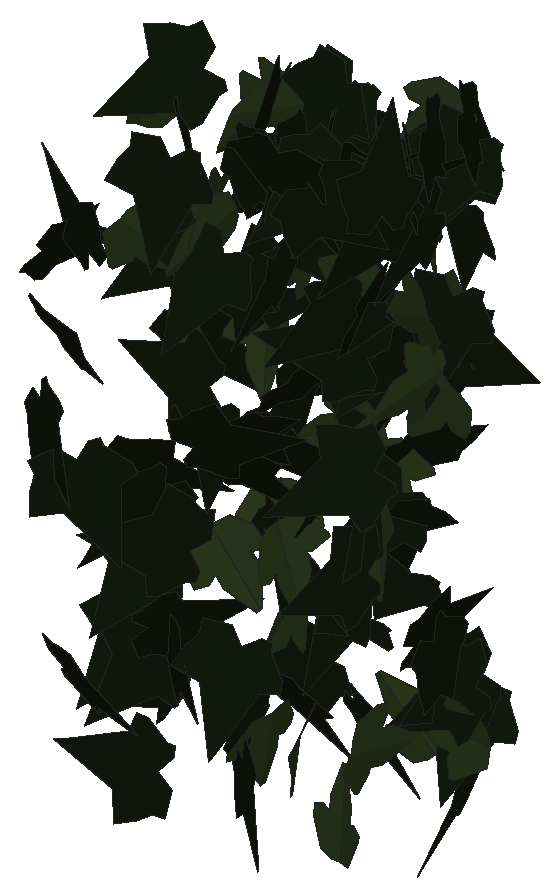
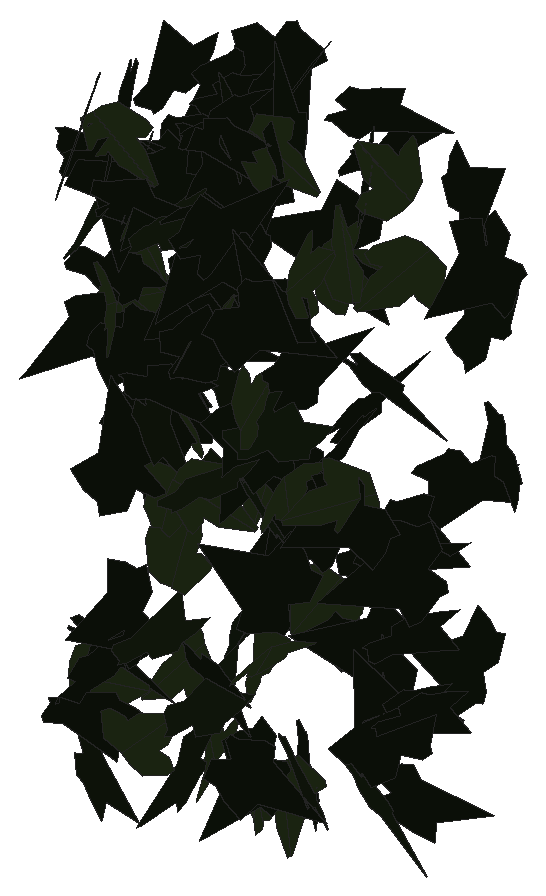
# SketchUp Ruby script. Lengths in inches.
U = 1.inch
M = Sketchup.active_model
def pt(a) = Geom::Point3d.new(a.map { |v| v * U })
def face(e, loops, mat)
  f = e.add_face(loops[0].map { |a| pt(a) })
  loops[1..].each { |l| e.add_face(l.map { |a| pt(a) }).erase! }
  f.material = f.back_material = mat if mat
  f
end
# faces: each face lists its corners as indices into pts; further lists are holes
def faces(e, pts, list, mat = nil) = list.each { |f| face(e, (f[0].is_a?(Array) ? f : [f]).map { |l| l.map { |i| pts[i] } }, mat) }
# xy, xz, yz: faces in a plane at the given z, y or x. An outline is a flat list of corners, or four numbers for a rectangle; further outlines are holes
def ring(l) = l.size == 4 ? [[l[0], l[1]], [l[2], l[1]], [l[2], l[3]], [l[0], l[3]]] : l.each_slice(2).to_a
def flat(e, list, mat, &to3) = list.each { |f| face(e, (f[0].is_a?(Array) ? f : [f]).map { |l| ring(l).map { |u, v| to3.(u, v) } }, mat) }
def xy(e, z, list, mat = nil) = flat(e, list, mat) { |x, y| [x, y, z] }
def xz(e, y, list, mat = nil) = flat(e, list, mat) { |x, z| [x, y, z] }
def yz(e, x, list, mat = nil) = flat(e, list, mat) { |y, z| [x, y, z] }
def lines(e, pts, list) = list.each { |a, b| e.add_line(pt(pts[a]), pt(pts[b])) }
# prism: a flat outline (further loops are holes) pulled along v
def prism(e, loops, v, mat = nil)
  f = face(e, loops, mat); d = Geom::Vector3d.new(v.map { |x| x * U })
  f.pushpull(f.normal.samedirection?(d) ? d.length : -d.length)
end
def box(e, o, s, mat = nil) = prism(e, [[o, [o[0] + s[0], o[1], o[2]], [o[0] + s[0], o[1] + s[1], o[2]], [o[0], o[1] + s[1], o[2]]]], [0, 0, s[2]], mat)
def at(x, y, z, deg = 0) = Geom::Transformation.translation(pt([x, y, z])) * Geom::Transformation.rotation(ORIGIN, Z_AXIS, deg.degrees)
def axes(o, x, y, z) = Geom::Transformation.new([*x, 0, *y, 0, *z, 0, *pt(o).to_a, 1])
def part(name) = M.definitions.add(name)
# library, detail: a bought-in or finely detailed component or shape, given as its bounding box
def library(name, o, s) = part(name).tap { |d| box(d.entities, o, s) }
def detail(e, o, s) = box(e.add_group.entities, o, s)
def put(e, d, t, mat = nil) = e.add_instance(d, t).tap { |i| i.material = mat if mat }
def group(e, t, mat = nil) = e.add_group.tap { |g| g.transformation = t; g.material = mat if mat }.entities
root = M.entities
M.materials.add("efeu1").color = [18, 25, 13]
M.materials.add("efeu2").color = [43, 57, 29]
c1 = part("ivyleaf_9")
p = [[1.54,2.16,1.25],[1.36,2.04,1.19],[-0.21,0.99,0.68],[-0.71,1.11,0.82],[-0.85,0.86,0.67],[-0.8,0.17,0.21],
  [-0.9,-0.01,0.1],[-0.67,-0.16,-0.02],[-0.08,-0.08,-0.05],[-0.03,-0.6,-0.4],[0.65,-0.88,-0.66],[0.83,-0.6,-0.49],
  [1.29,-0.42,-0.43],[1.8125,-0.07,-0.26],[1.21,0.44,0.15]]
faces(c1.entities,p,[[0,1,2,3,4,5,6,7,8,9,10,11,12,13,14]],"efeu1")
c2 = part("ivyleaf_10")
p = [[0,0.5,-0.03],[-0.0625,2.02,-0.43],[-0.19,2.01,-0.46],[-0.54,1.05,-0.29],[-0.52,0.625,-0.18],[-0.83,0.76,-0.28],
  [-1.16,0.64,-0.33],[-1.15,0.33,-0.24],[-0.77,-0.39,0.02],[-0.3,-0.51,0.16],[0.04,-0.48,0.23],[-0.02,2.01,-0.4375],
  [-0.06,2.01,-0.43],[0.04,-0.49,0.23],[0.67,-0.49,0.14],[1.38,0.36,-0.2],[1.375,0.51,-0.24],[0.81,0.65,-0.19],
  [0.62,0.59,-0.15],[0.6,1.09,-0.28],[0.5,1.23,-0.31]]
faces(c2.entities,p,[[0,1,2,3,4,5,6,7,8,9,10],[11,12,0,13,14,15,16,17,18,19,20]],"efeu2")
put(root,c1,axes([51.28,217.17,229.75],[0.22094,-0.00103,0.44854],[0.44724,0.03852,-0.22021],[-0.0341,0.49851,0.01794]))
put(root,c1,axes([48.23,218.1,229.92],[0.44307,-0.12316,-0.19627],[0.1976,-0.02037,0.45885],[-0.12102,-0.48417,0.03062]))
put(root,c1,axes([48.84,217.92,231.51],[0.08057,-0.14995,0.47013],[-0.25668,0.39411,0.16969],[-0.42145,-0.26869,-0.01347]))
put(root,c1,axes([48.23,218.3,224.89],[0.3039,-0.23486,0.32013],[0.24876,-0.20158,-0.38403],[0.30946,0.39269,-0.00567]))
put(root,c1,axes([47.69,218.4375,228.55],[-0.0903,-0.03685,-0.4904],[0.49111,0.01929,-0.09188],[0.02569,-0.49827,0.03271]))
put(root,c1,axes([48.37,218.33,227.95],[-0.12204,-0.31328,-0.37009],[0.14117,0.34214,-0.33617],[0.46387,-0.18654,0.00495]))
put(root,c1,axes([48.05,218.09,231.11],[0.1964,0.32583,0.32444],[0.17294,0.27456,-0.38041],[-0.42605,0.26164,-0.00485]))
put(root,c1,axes([49.52,218.77,232.61],[-0.14679,-0.47709,-0.02902],[0.00927,0.02751,-0.49916],[0.47788,-0.14708,0.00076]))
put(root,c1,axes([51.42,218.64,233.4375],[0.22565,0.22473,-0.38546],[-0.28444,-0.26034,-0.3183],[-0.34377,0.36293,0.01035]))
put(root,c1,axes([50.82,218.66,233.26],[0.32245,-0.23472,-0.30156],[-0.17593,0.25909,-0.38977],[0.33923,0.35747,0.0845]))
put(root,c1,axes([52.62,218.9,227.59],[-0.46595,0.14301,0.11152],[-0.10762,0.02941,-0.48739],[-0.14597,-0.47821,0.00337]))
put(root,c1,axes([52.4375,219.24,228.87],[-0.39221,-0.16195,0.26447],[-0.24473,-0.10025,-0.42433],[0.19047,-0.4623,-0.00063]))
put(root,c1,axes([50.27,219.27,225.45],[-0.35521,-0.31837,-0.14989],[0.12497,0.08496,-0.47662],[0.32895,-0.37606,0.01922]))
put(root,c1,axes([48.87,219.42,227.27],[-0.08262,0.06028,-0.48943],[0.11063,-0.48134,-0.07796],[-0.48056,-0.12117,0.06619]))
put(root,c1,axes([51.8,218.86,232.96],[0.06545,-0.16299,-0.46813],[-0.06779,0.46482,-0.17132],[0.49104,0.08589,0.03875]))
put(root,c1,axes([49.1,219.34,225.17],[0.0759,-0.08251,-0.48727],[0.49079,-0.04532,0.08412],[-0.05805,-0.49106,0.07411]))
put(root,c1,axes([51.66,219.46,232.93],[-0.35236,-0.30007,0.18922],[-0.13499,-0.13322,-0.46263],[0.32806,-0.37711,0.01287]))
put(root,c1,axes([48.89,219.24,223.22],[-0.26142,-0.13816,-0.4032],[-0.31821,-0.25141,0.29246],[-0.28355,0.40952,0.04352]))
put(root,c1,axes([49.23,219.47,226.5],[-0.15309,-0.06751,0.47117],[-0.43495,-0.18121,-0.16729],[0.19334,-0.46109,-0.00324]))
put(root,c2,axes([48.72,219.07,231.24],[-0.29511,-0.1897,-0.35626],[0.32293,0.15378,-0.34938],[0.24213,-0.43631,0.03175]))
put(root,c2,axes([51.08,219.17,227.41],[0.06416,0.4922,0.06023],[0.00954,0.0595,-0.49636],[-0.49577,0.06484,-0.00176]))
put(root,c1,axes([49.78,219.49,230.99],[-0.43714,-0.23622,-0.05576],[0.04885,0.0269,-0.49688],[0.23774,-0.43986,-0.00044]))
put(root,c1,axes([49.35,219.59,233.5625],[-0.38786,-0.17449,0.2629],[-0.23968,-0.10802,-0.4253],[0.20522,-0.45595,0.00015]))
put(root,c1,axes([51.91,219.02,228.42],[-0.11774,0.42278,0.23958],[-0.06777,0.22982,-0.43885],[-0.48119,-0.13581,0.00319]))
put(root,c1,axes([48.64,219.6875,224.73],[-0.28187,-0.35334,0.21378],[-0.11764,-0.17941,-0.45163],[0.39587,-0.3049,0.01801]))
put(root,c1,axes([51.02,219.6875,233.06],[0.04465,-0.04359,-0.49609],[0.31833,-0.38054,0.06209],[-0.38298,-0.32139,-0.00623]))
put(root,c2,axes([52.27,219.56,227.95],[0.37124,-0.15212,0.2984],[0.2756,-0.11439,-0.4012],[0.19033,0.46236,-0.00108]))
put(root,c1,axes([49.36,219.72,228.86],[-0.01401,-0.48605,-0.11644],[0.0059,-0.11664,0.48617],[-0.49977,0.01225,0.00901]))
put(root,c1,axes([49.49,219.78,228.47],[0.02418,-0.47675,0.14874],[0.00401,-0.14873,-0.47735],[0.4994,0.02427,-0.00337]))
put(root,c1,axes([48.4375,219.83,226.03],[-0.26894,-0.38758,0.16568],[-0.07717,-0.14794,-0.47134],[0.41439,-0.27909,0.01976]))
put(root,c1,axes([52.54,219.37,232.7],[-0.18468,-0.28157,0.36961],[0.23871,0.28374,0.33543],[-0.39864,0.30035,0.02962]))
put(root,c1,axes([50,219.7,223.48],[-0.09719,-0.0126,-0.4903],[0.48809,-0.05161,-0.09543],[-0.04821,-0.49717,0.02234]))
put(root,c1,axes([48.27,219.86,224.89],[-0.28744,-0.37434,0.16507],[-0.09017,-0.13881,-0.4718],[0.39906,-0.301,0.01229]))
put(root,c2,axes([49.45,219.9,231.24],[0.01634,-0.19906,0.45838],[0.03995,-0.45663,-0.19972],[0.49813,0.04315,0.00098]))
put(root,c1,axes([48.9,219.23,225.34],[0.15349,0.34314,-0.32969],[0.08944,0.31944,0.37411],[0.46738,-0.17382,0.03668]))
put(root,c1,axes([52.38,219.92,228.21],[-0.18405,-0.41917,0.20105],[-0.07748,-0.18555,-0.45778],[0.45839,-0.19966,0.00335]))
put(root,c1,axes([48.9375,219.88,232.43],[-0.08237,0.06218,0.48923],[0.017,-0.49536,0.06582],[0.49288,0.02748,0.07949]))
put(root,c1,axes([52.18,220.0625,232.23],[-0.02253,0.10528,-0.48827],[0.09145,-0.47964,-0.10763],[-0.49105,-0.09415,0.00235]))
put(root,c2,axes([48.54,219.65,232.67],[-0.00537,-0.43402,0.24819],[0.02328,0.24772,0.4337],[-0.49943,0.01622,0.01755]))
put(root,c2,axes([49.13,220,231.2],[0.08054,-0.44388,-0.2156],[0.08788,-0.20206,0.44883],[-0.48558,-0.11019,0.04546]))
put(root,c1,axes([48.34,219.89,224.35],[0.45686,0.20313,0.0038],[-0.00611,0.00438,0.49994],[0.20308,-0.45686,0.00649]))
put(root,c1,axes([52.43,219.66,228.06],[0.2672,0.40187,-0.13079],[-0.07714,-0.10577,-0.48256],[-0.41552,0.27805,0.00548]))
put(root,c1,axes([50.1,219.96,232.84],[0.03033,0.35186,0.35394],[-0.07222,-0.34777,0.35191],[0.49383,-0.07247,0.02973]))
put(root,c2,axes([52.6,220.27,229.85],[0.0043,-0.08835,0.49211],[0.03392,-0.49095,-0.08844],[0.49883,0.03415,0.00177]))
put(root,c2,axes([51.62,219.61,222.97],[-0.02133,0.37206,-0.33334],[-0.06627,0.32859,0.37099],[0.49513,0.06001,0.03529]))
put(root,c2,axes([51.97,219.67,224.43],[-0.05649,-0.13484,-0.47815],[0.13835,0.45792,-0.14548],[0.47714,-0.14875,-0.01443]))
put(root,c2,axes([49.42,219.92,226.46],[0.32909,0.2475,0.28363],[0.22931,0.16696,-0.41175],[-0.29853,0.40108,-0.00362]))
put(root,c1,axes([51.37,220.33,230.47],[-0.02592,0.04935,-0.49688],[-0.08027,-0.49149,-0.04463],[-0.49283,0.07746,0.0334]))
put(root,c1,axes([47.97,219.83,227.2],[0.39956,0.10916,0.28007],[0.27234,0.06572,-0.41414],[-0.12722,0.48349,-0.00694]))
put(root,c1,axes([51.22,219.75,232.67],[0.00238,0.09641,0.49061],[-0.03172,0.48966,-0.09607],[-0.49899,-0.03067,0.00845]))
put(root,c1,axes([50.89,219.96,232.24],[0.12964,0.45867,-0.15106],[-0.0609,-0.13963,-0.47623],[-0.47904,0.14188,0.01967]))
put(root,c1,axes([50.28,220.25,230.77],[-0.40523,0.19883,-0.21506],[0.18411,-0.11261,-0.45103],[-0.22779,-0.44473,0.01805]))
put(root,c1,axes([51.46,220.33,229.74],[-0.22761,-0.00013,0.44519],[-0.44435,-0.03068,-0.22719],[0.02737,-0.49906,0.01385]))
put(root,c1,axes([52.61,220.3,232.23],[-0.44601,0.14653,-0.17205],[0.1616,-0.05931,-0.46943],[-0.15798,-0.47435,0.00555]))
put(root,c2,axes([52.58,220.15,230.83],[-0.20171,0.02213,0.45697],[-0.45132,0.07224,-0.20272],[-0.07499,-0.49426,-0.00916]))
put(root,c1,axes([49.44,220.08,227.62],[0.4821,0.06994,0.11266],[0.11164,0.01515,-0.48714],[-0.07156,0.49485,-0.00101]))
put(root,c2,axes([50.29,220.33,233.04],[-0.19507,-0.04407,0.45826],[-0.43929,-0.13109,-0.1996],[0.13774,-0.48049,0.01242]))
put(root,c1,axes([49.54,220,228.09],[0.31498,0.38024,0.07875],[0.0392,0.06974,-0.49356],[-0.38633,0.3171,0.01412]))
put(root,c1,axes([50.875,220.69,233.36],[-0.18768,-0.43628,0.15632],[-0.03977,-0.15287,-0.47439],[0.46173,-0.1905,0.02268]))
put(root,c2,axes([50.08,220.68,225.52],[-0.00465,0.17553,-0.46815],[0.00183,-0.46816,-0.17555],[-0.49998,-0.00335,0.00371]))
put(root,c1,axes([48.46,220.46,230.33],[-0.49097,0.06112,0.07217],[-0.07168,0.00839,-0.49476],[-0.06169,-0.49618,0.00052]))
put(root,c2,axes([52.75,220.39,229.62],[-0.38972,-0.0207,0.31256],[-0.30644,-0.07823,-0.38727],[0.06494,-0.49341,0.04829]))
put(root,c1,axes([49.9,220.75,226.35],[0.06385,-0.39855,0.29509],[0.04545,-0.29157,-0.40363],[0.49382,0.07837,-0.00101]))
put(root,c1,axes([49.49,220.82,229.85],[-0.08068,-0.08752,0.48562],[-0.34578,-0.34102,-0.11891],[0.35203,-0.35503,-0.0055]))
put(root,c1,axes([48.45,220.42,224.04],[-0.37768,0.32046,0.06828],[-0.05403,0.04186,-0.49531],[-0.32317,-0.38151,0.00301]))
put(root,c2,axes([49.77,220.5,223.65],[-0.03581,-0.4973,-0.03754],[0.00819,0.03704,-0.49856],[0.49865,-0.03633,0.00549]))
put(root,c2,axes([50.05,220.83,223.375],[-0.01569,-0.15992,-0.47348],[0.1375,-0.45681,0.14973],[-0.48047,-0.12551,0.05831]))
put(root,c1,axes([50.08,220.87,226.12],[0.31269,-0.31986,-0.22341],[0.1734,-0.14254,0.44678],[-0.3495,-0.35689,0.02178]))
put(root,c1,axes([49.7,220.29,223.8],[-0.31155,0.13313,-0.36772],[-0.34547,0.12664,0.33855],[0.18328,0.46501,0.01308]))
put(root,c1,axes([50.82,220.82,233.26],[-0.45673,-0.20196,-0.02472],[0.01804,0.0203,-0.49926],[0.20267,-0.45695,-0.01126]))
put(root,c1,axes([52.52,220.83,230.72],[-0.37264,-0.27232,-0.19231],[0.15508,0.11372,-0.46154],[0.29511,-0.40362,-0.00029]))
put(root,c2,axes([51.27,220.96,226.5625],[-0.12007,-0.36805,-0.31642],[-0.04654,-0.31572,0.38491],[-0.48313,0.12189,0.04156]))
put(root,c1,axes([51.45,220.28,230.375],[-0.13023,0.24547,-0.41567],[-0.27106,0.31908,0.27335],[0.39946,0.29653,0.04997]))
put(root,c1,axes([52.41,220.49,233.34],[0.18176,-0.11752,-0.45072],[-0.39084,0.22472,-0.2162],[0.2534,0.43091,-0.01017]))
put(root,c1,axes([49.9,220.83,231.58],[0.10205,0.02378,-0.4889],[0.48738,0.04117,0.10374],[0.04519,-0.49773,-0.01478]))
put(root,c1,axes([52.08,220.96,229.85],[0.0452,0.08385,-0.49084],[-0.28017,-0.40317,-0.09467],[-0.41166,0.28359,0.01054]))
put(root,c1,axes([51.51,220.47,232.2],[0.20396,0.38176,0.25032],[0.09588,0.23223,-0.43229],[-0.44633,0.22434,0.02153]))
put(root,c1,axes([50.14,220.51,228.82],[0.17163,0.44488,0.15043],[0.02465,0.15141,-0.47589],[-0.46897,0.17076,0.03004]))
put(root,c1,axes([52.74,220.96,225.04],[-0.47756,0.0765,0.12681],[-0.12525,0.01988,-0.48365],[-0.07904,-0.49371,0.00018]))
put(root,c1,axes([52.18,220.85,231.64],[0.05154,-0.38064,0.32008],[0.00943,0.32249,0.38199],[-0.49725,-0.03334,0.04042]))
put(root,c2,axes([52.82,220.86,224.33],[-0.05062,0.03332,-0.49631],[-0.48763,0.09522,0.05613],[0.09826,0.48972,0.02285]))
put(root,c1,axes([52.35,220.73,225.63],[0.17803,-0.23759,-0.40231],[-0.25572,0.31077,-0.2967],[0.39104,0.3114,-0.01086]))
put(root,c1,axes([49.8,220.82,224.08],[0.49644,-0.01102,-0.05852],[-0.05845,0.00388,-0.49656],[0.01139,0.49986,0.00256]))
put(root,c2,axes([51.92,220.93,231.91],[-0.25215,0.43139,-0.01799],[0.00913,-0.0155,-0.49968],[-0.43167,-0.25232,-0.00006]))
put(root,c2,axes([51.24,220.97,227.86],[0.42761,0.2214,0.13465],[0.09747,0.10331,-0.4794],[-0.2401,0.43624,0.04519]))
put(root,c1,axes([52.32,221.3,232.63],[-0.32124,-0.38311,0.00555],[-0.00168,-0.00584,-0.49996],[0.38315,-0.32124,0.00247]))
put(root,c1,axes([52.46,221.27,232.81],[-0.42874,-0.24883,-0.06534],[0.04856,0.04643,-0.49547],[0.25264,-0.43119,-0.01565]))
put(root,c1,axes([52.13,220.87,232.38],[0.15783,0.46265,-0.1051],[-0.03424,-0.09936,-0.48883],[-0.4732,0.1615,0.00031]))
put(root,c2,axes([50.73,221.26,230.02],[-0.13321,0.37957,0.29696],[0.01869,-0.30379,0.39669],[0.48157,0.11678,0.06674]))
put(root,c2,axes([48.77,221.4375,231.93],[0.00679,0.0043,0.49994],[0.21023,-0.45365,0.00105],[0.4536,0.21019,-0.00796]))
put(root,c2,axes([52.1,221.3,230.43],[-0.21438,0.18297,-0.41299],[0.22171,-0.35567,-0.27266],[-0.39356,-0.30003,0.07137]))
put(root,c1,axes([50.52,221.25,225.49],[-0.46219,-0.02125,-0.18955],[0.18921,0.01173,-0.46267],[0.02411,-0.49941,-0.0028]))
put(root,c1,axes([49.78,221.23,228.375],[-0.44646,0.15118,-0.16678],[0.1537,-0.06593,-0.4712],[-0.16446,-0.47202,0.0124]))
put(root,c1,axes([52.45,221.34,223.45],[-0.34945,0.15136,-0.324],[0.25945,-0.20446,-0.37534],[-0.24612,-0.43045,0.06436]))
put(root,c1,axes([52.02,220.76,225.54],[0.11436,0.19947,0.444],[0.20718,0.39276,-0.22981],[-0.44045,0.23654,0.00718]))
put(root,c1,axes([52.2,221.5,231.68],[0.0623,-0.41341,0.27425],[0.07048,-0.26623,-0.41732],[0.49107,0.09066,0.0251]))
put(root,c1,axes([51.46,221.25,229],[-0.35141,0.27998,-0.21937],[0.16618,-0.14341,-0.44924],[-0.31448,-0.38864,0.00774]))
put(root,c1,axes([51.28,221.42,229.62],[-0.4387,-0.23955,0.01264],[-0.01123,-0.00579,-0.49984],[0.23962,-0.43884,-0.0003]))
put(root,c2,axes([50.75,221.23,228.07],[0.20623,0.02032,-0.45503],[-0.45529,0.02408,-0.20527],[0.01358,0.49901,0.02843]))
put(root,c1,axes([49.18,221.57,229.39],[-0.22297,-0.4255,0.13868],[0.35349,-0.26247,-0.23697],[0.27446,-0.00763,0.41787]))
put(root,c1,axes([50.32,221.51,231.93],[0.00785,-0.00618,0.4999],[-0.41187,-0.28347,0.00297],[0.28337,-0.41184,-0.00954]))
put(root,c1,axes([52.38,220.89,229.96],[0.09927,-0.04066,-0.48836],[-0.0319,0.49668,-0.04784],[0.48901,0.04065,0.09602]))
put(root,c1,axes([52.35,221.62,224.78],[-0.17833,-0.28208,0.37233],[-0.1878,-0.32162,-0.33361],[0.4277,-0.25883,0.00876]))
put(root,c1,axes([50.7,221.19,223.95],[0.4154,-0.26028,-0.09845],[-0.07871,0.05976,-0.49014],[0.26692,0.42271,0.00868]))
put(root,c1,axes([47.97,221.14,228.72],[-0.03965,-0.04294,-0.49657],[0.3411,0.36088,-0.05844],[0.36342,-0.3434,0.00068]))
put(root,c2,axes([51.73,221.28,223.82],[0.35224,0.12483,0.33218],[-0.30906,-0.1221,0.3736],[0.17439,-0.46852,-0.00886]))
put(root,c1,axes([49.29,221.22,231.08],[-0.28624,0.14941,0.38177],[0.31174,-0.22306,0.32103],[0.26624,0.42181,0.03454]))
put(root,c2,axes([48.91,221.52,228.83],[-0.11584,-0.42424,0.23792],[0.27237,-0.25921,-0.32959],[0.40299,0.05324,0.29115]))
put(root,c1,axes([50.9,221.7,231.98],[-0.30622,-0.32283,0.22806],[0.17543,-0.36952,-0.28754],[0.3542,-0.09608,0.33958]))
put(root,c1,axes([49.88,221.41,224.29],[-0.06449,-0.02086,-0.49538],[-0.365,-0.33611,0.06167],[-0.33558,0.36958,0.02813]))
put(root,c1,axes([51.86,221.49,232.09],[-0.35761,-0.01123,0.34927],[-0.34668,-0.05136,-0.35661],[0.04389,-0.49723,0.02895]))
put(root,c1,axes([52.54,221.1,233.34],[0.25968,-0.1131,-0.41204],[-0.35109,0.21831,-0.2812],[0.24351,0.43537,0.03397]))
put(root,c1,axes([51.61,221.38,227.89],[0.3371,0.30885,0.20241],[-0.14661,-0.1396,0.45718],[0.33892,-0.36759,-0.00356]))
put(root,c1,axes([50.34,221.12,231.98],[0.47058,0.16654,-0.02869],[-0.02583,-0.01303,-0.49916],[-0.16701,0.47127,-0.00366]))
put(root,c1,axes([50.3,221.73,224.91],[-0.30774,-0.26479,0.29186],[0.17685,-0.42372,-0.19796],[0.35217,-0.01861,0.35444]))
put(root,c1,axes([50.55,221.64,230.34],[-0.17715,-0.1056,0.45548],[-0.40895,-0.20112,-0.20569],[0.22666,-0.44542,-0.01511]))
put(root,c2,axes([52.0625,221.37,233.17],[0.37873,-0.00642,-0.32638],[-0.3247,0.04408,-0.37766],[0.03362,0.49801,0.02922]))
put(root,c1,axes([51.05,221.78,225.77],[-0.24361,-0.35862,0.24909],[0.19622,-0.34473,-0.3044],[0.39006,-0.05055,0.3087]))
put(root,c2,axes([49.12,221.62,226.27],[-0.2228,-0.43201,0.11714],[0.35317,-0.25006,-0.25049],[0.27501,-0.02888,0.41657]))
put(root,c2,axes([48.05,221.13,228.82],[0.08064,0.10468,0.48222],[0.26882,0.40043,-0.13188],[-0.4138,0.28053,0.0083]))
put(root,c1,axes([49.53,221.67,231.39],[-0.04425,0.05287,-0.49522],[-0.09893,-0.4882,-0.04328],[-0.48811,0.09415,0.05367]))
put(root,c1,axes([50.16,221.79,228.42],[-0.14352,-0.4299,0.21115],[0.22905,-0.25519,-0.36389],[0.42064,-0.00772,0.27018]))
put(root,c1,axes([52.28,221.64,224.42],[-0.35659,-0.33191,-0.11262],[0.08186,0.07734,-0.48715],[0.3408,-0.36586,-0.00081]))
put(root,c1,axes([49,221.46,227.07],[0.14955,-0.14811,0.45354],[0.44548,-0.12683,-0.18831],[0.17083,0.46041,0.09403]))
put(root,c2,axes([49.37,221.85,229.9],[-0.00978,-0.09567,-0.49066],[0.01247,-0.49065,0.09542],[-0.49975,-0.01037,0.01198]))
